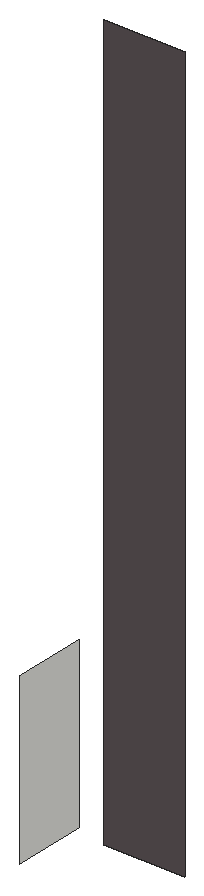
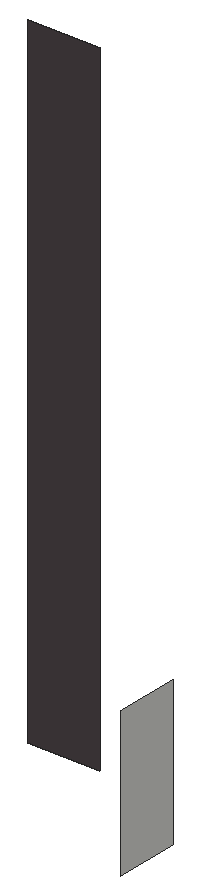
# SketchUp Ruby script. Lengths in inches.
U = 1.inch
M = Sketchup.active_model
def pt(a) = Geom::Point3d.new(a.map { |v| v * U })
def face(e, loops, mat)
  f = e.add_face(loops[0].map { |a| pt(a) })
  loops[1..].each { |l| e.add_face(l.map { |a| pt(a) }).erase! }
  f.material = f.back_material = mat if mat
  f
end
# faces: each face lists its corners as indices into pts; further lists are holes
def faces(e, pts, list, mat = nil) = list.each { |f| face(e, (f[0].is_a?(Array) ? f : [f]).map { |l| l.map { |i| pts[i] } }, mat) }
# xy, xz, yz: faces in a plane at the given z, y or x. An outline is a flat list of corners, or four numbers for a rectangle; further outlines are holes
def ring(l) = l.size == 4 ? [[l[0], l[1]], [l[2], l[1]], [l[2], l[3]], [l[0], l[3]]] : l.each_slice(2).to_a
def flat(e, list, mat, &to3) = list.each { |f| face(e, (f[0].is_a?(Array) ? f : [f]).map { |l| ring(l).map { |u, v| to3.(u, v) } }, mat) }
def xy(e, z, list, mat = nil) = flat(e, list, mat) { |x, y| [x, y, z] }
def xz(e, y, list, mat = nil) = flat(e, list, mat) { |x, z| [x, y, z] }
def yz(e, x, list, mat = nil) = flat(e, list, mat) { |y, z| [x, y, z] }
def lines(e, pts, list) = list.each { |a, b| e.add_line(pt(pts[a]), pt(pts[b])) }
# prism: a flat outline (further loops are holes) pulled along v
def prism(e, loops, v, mat = nil)
  f = face(e, loops, mat); d = Geom::Vector3d.new(v.map { |x| x * U })
  f.pushpull(f.normal.samedirection?(d) ? d.length : -d.length)
end
def box(e, o, s, mat = nil) = prism(e, [[o, [o[0] + s[0], o[1], o[2]], [o[0] + s[0], o[1] + s[1], o[2]], [o[0], o[1] + s[1], o[2]]]], [0, 0, s[2]], mat)
def at(x, y, z, deg = 0) = Geom::Transformation.translation(pt([x, y, z])) * Geom::Transformation.rotation(ORIGIN, Z_AXIS, deg.degrees)
def axes(o, x, y, z) = Geom::Transformation.new([*x, 0, *y, 0, *z, 0, *pt(o).to_a, 1])
def part(name) = M.definitions.add(name)
# library, detail: a bought-in or finely detailed component or shape, given as its bounding box
def library(name, o, s) = part(name).tap { |d| box(d.entities, o, s) }
def detail(e, o, s) = box(e.add_group.entities, o, s)
def put(e, d, t, mat = nil) = e.add_instance(d, t).tap { |i| i.material = mat if mat }
def group(e, t, mat = nil) = e.add_group.tap { |g| g.transformation = t; g.material = mat if mat }.entities
root = M.entities
M.materials.add("[Asphalt New]").color = [91, 82, 84]
xz(root,92.3,[[334.81,18.11,339.17,57.8125]],"[Asphalt New]")
yz(root,330.33,[[92.3,15.61,96.24,24.68]])
